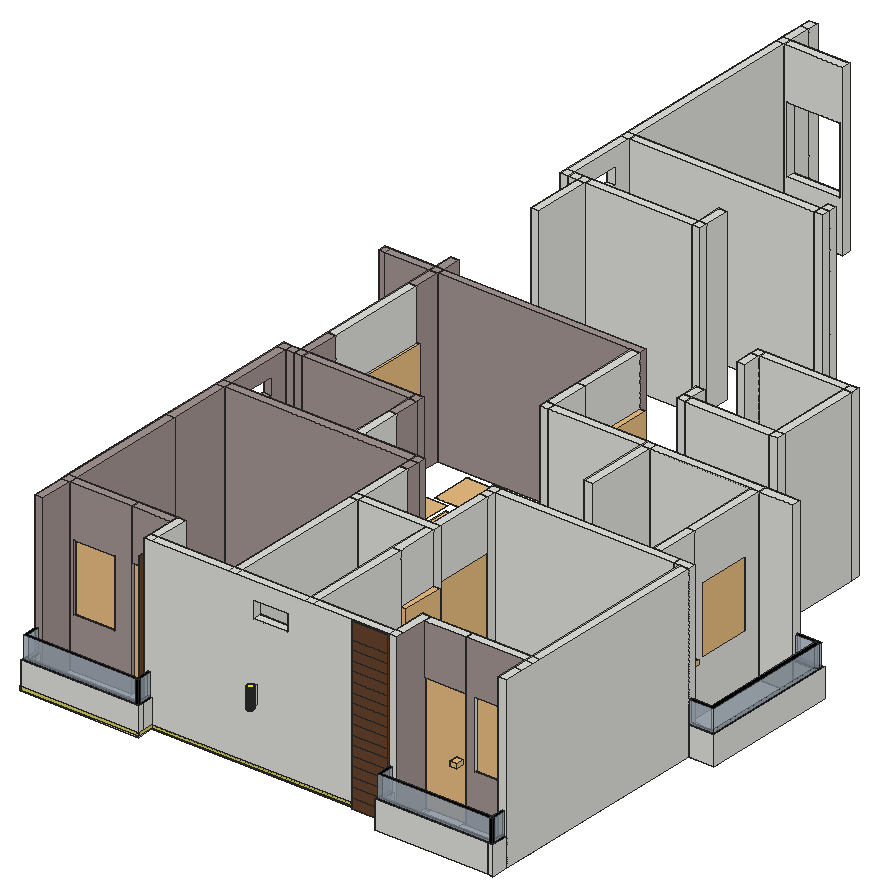
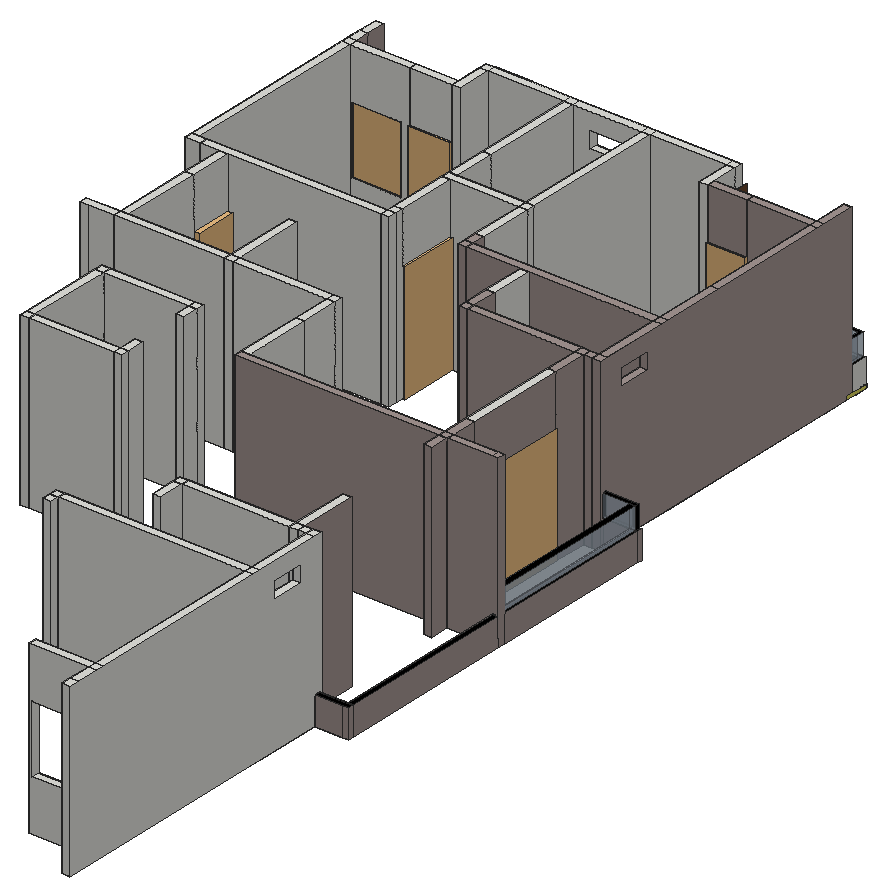
# SketchUp Ruby script. Lengths in inches.
U = 1.inch
M = Sketchup.active_model
def pt(a) = Geom::Point3d.new(a.map { |v| v * U })
def face(e, loops, mat)
  f = e.add_face(loops[0].map { |a| pt(a) })
  loops[1..].each { |l| e.add_face(l.map { |a| pt(a) }).erase! }
  f.material = f.back_material = mat if mat
  f
end
# faces: each face lists its corners as indices into pts; further lists are holes
def faces(e, pts, list, mat = nil) = list.each { |f| face(e, (f[0].is_a?(Array) ? f : [f]).map { |l| l.map { |i| pts[i] } }, mat) }
# xy, xz, yz: faces in a plane at the given z, y or x. An outline is a flat list of corners, or four numbers for a rectangle; further outlines are holes
def ring(l) = l.size == 4 ? [[l[0], l[1]], [l[2], l[1]], [l[2], l[3]], [l[0], l[3]]] : l.each_slice(2).to_a
def flat(e, list, mat, &to3) = list.each { |f| face(e, (f[0].is_a?(Array) ? f : [f]).map { |l| ring(l).map { |u, v| to3.(u, v) } }, mat) }
def xy(e, z, list, mat = nil) = flat(e, list, mat) { |x, y| [x, y, z] }
def xz(e, y, list, mat = nil) = flat(e, list, mat) { |x, z| [x, y, z] }
def yz(e, x, list, mat = nil) = flat(e, list, mat) { |y, z| [x, y, z] }
def lines(e, pts, list) = list.each { |a, b| e.add_line(pt(pts[a]), pt(pts[b])) }
# prism: a flat outline (further loops are holes) pulled along v
def prism(e, loops, v, mat = nil)
  f = face(e, loops, mat); d = Geom::Vector3d.new(v.map { |x| x * U })
  f.pushpull(f.normal.samedirection?(d) ? d.length : -d.length)
end
def box(e, o, s, mat = nil) = prism(e, [[o, [o[0] + s[0], o[1], o[2]], [o[0] + s[0], o[1] + s[1], o[2]], [o[0], o[1] + s[1], o[2]]]], [0, 0, s[2]], mat)
def at(x, y, z, deg = 0) = Geom::Transformation.translation(pt([x, y, z])) * Geom::Transformation.rotation(ORIGIN, Z_AXIS, deg.degrees)
def axes(o, x, y, z) = Geom::Transformation.new([*x, 0, *y, 0, *z, 0, *pt(o).to_a, 1])
def part(name) = M.definitions.add(name)
# library, detail: a bought-in or finely detailed component or shape, given as its bounding box
def library(name, o, s) = part(name).tap { |d| box(d.entities, o, s) }
def detail(e, o, s) = box(e.add_group.entities, o, s)
def put(e, d, t, mat = nil) = e.add_instance(d, t).tap { |i| i.material = mat if mat }
def group(e, t, mat = nil) = e.add_group.tap { |g| g.transformation = t; g.material = mat if mat }.entities
root = M.entities
M.materials.add("2121 AP  X165 Dhaani-I").color = [217, 210, 92]
M.materials.add("Glass_Basic_01").color = [161, 173, 186]
M.materials["Glass_Basic_01"].alpha = 0.59
M.materials.add("M09_Shadow_Night").color = [0, 0, 0]
M.materials.add("Marble_06_1K").color = [165, 150, 147]
M.materials.add("Wood_Veneer_15_1K").color = [103, 69, 45]
M.materials.add("[0056_Yellow]").color = [255, 255, 0]
c1 = part("Group\#8")
xy(c1.entities,0,[[0,-8.88,4,-4.88],[4,-8.88,80,-4.88],[80,-8.88,84,-4.88],[0,-4.88,4,0],[80,-4.88,84,3.12],
  [0,0,4,3.12]])
xy(c1.entities,20,[[0,-8.88,4,-4.88],[4,-8.88,80,-4.88],[80,-8.88,84,-4.88],[0,-4.88,4,0],[80,-4.88,84,3.12],
  [0,0,4,3.12]],"M09_Shadow_Night")
xz(c1.entities,-8.88,[[0,0,80,20],[80,0,84,20]])
xz(c1.entities,-4.88,[[4,0,80,20]])
xz(c1.entities,3.12,[[0,0,4,20],[80,0,84,20]])
yz(c1.entities,0,[[-8.88,0,3.12,20]])
yz(c1.entities,4,[[-4.88,0,0,20],[0,0,3.12,20]])
yz(c1.entities,80,[[-8.88,0,-4.88,20],[-4.88,0,3.12,20]])
yz(c1.entities,84,[[-8.88,0,3.12,20]])
c2 = part("Group\#6")
xy(c2.entities,0,[[0,-8,80,-4],[80,-8,84,-4],[0,-4,4,0],[80,-4,84,4],[0,0,4,4]])
xy(c2.entities,20,[[0,-8,84,-8,84,4,80,4,80,-4,4,-4,4,4,0,4]],"M09_Shadow_Night")
xz(c2.entities,-8,[[0,0,84,20]])
xz(c2.entities,-4,[[4,0,80,20]])
xz(c2.entities,4,[[0,0,4,20],[80,0,84,20]])
yz(c2.entities,0,[[-8,0,4,20]])
yz(c2.entities,4,[[-4,0,0,20],[0,0,4,20]])
yz(c2.entities,80,[[-4,0,4,20]])
yz(c2.entities,84,[[-8,0,-4,20],[-4,0,4,20]])
c3 = part("Group\#87")
xy(c3.entities,0,[[0,0,0,11.0625,2,11.0625,2,2,80,2,80,0],[80,0,82,2],[80,2,82,11.0625]])
xy(c3.entities,16,[[0,0,80,0,80,2,2,2,2,11.0625,0,11.0625],[80,0,82,2],[80,2,82,11.0625]],"M09_Shadow_Night")
xz(c3.entities,0,[[0,0,80,16]],"Glass_Basic_01")
xz(c3.entities,0,[[80,0,82,16]],"M09_Shadow_Night")
xz(c3.entities,2,[[2,0,80,16],[80,0,82,16]])
xz(c3.entities,11.0625,[[0,0,2,16],[80,0,82,16]])
yz(c3.entities,0,[[0,0,11.0625,16]])
yz(c3.entities,2,[[2,0,11.0625,16]])
yz(c3.entities,80,[[0,0,2,16],[2,0,11.0625,16]])
yz(c3.entities,82,[[2,0,11.0625,16]])
yz(c3.entities,82,[[0,0,2,16]],"M09_Shadow_Night")
c4 = part("Group\#89")
xy(c4.entities,0,[[0,0,0,11.0625,2,11.0625,2,2,80,2,80,0],[80,0,82,2],[80,2,82,11.0625]])
xy(c4.entities,16,[[0,0,80,0,80,2,2,2,2,11.0625,0,11.0625],[80,0,82,2],[80,2,82,11.0625]],"M09_Shadow_Night")
xz(c4.entities,0,[[0,0,80,16]],"Glass_Basic_01")
xz(c4.entities,0,[[80,0,82,16]],"M09_Shadow_Night")
xz(c4.entities,2,[[2,0,80,16],[80,0,82,16]])
xz(c4.entities,11.0625,[[0,0,2,16],[80,0,82,16]])
yz(c4.entities,0,[[0,0,11.0625,16]])
yz(c4.entities,2,[[2,0,11.0625,16]])
yz(c4.entities,80,[[0,0,2,16],[2,0,11.0625,16]])
yz(c4.entities,82,[[2,0,11.0625,16]])
yz(c4.entities,82,[[0,0,2,16]],"M09_Shadow_Night")
c5 = part("Wall light")
xy(c5.entities,0,[[1.3,1.93,0.875,2.1,0.51,2.38,0.23,2.74,0.06,3.17,0,3.62,0.06,4.07,0.23,4.49,0.51,4.86,0.875,5.13,1.3,5.31,1.75,5.37,2.2,5.31,2.625,5.13,2.99,4.86,3.27,4.49,3.44,4.07,3.5,3.62,3.44,3.17,3.27,2.74,2.99,2.38,2.625,2.1,2.2,1.93]],"[0056_Yellow]")
xy(c5.entities,0.74,[[1.01,0,2.57,1.93]])
xy(c5.entities,10.13,[[1.01,0,2.57,0,2.57,1.93,2.2,1.93,1.75,1.87,1.3,1.93,1.01,1.93]])
xy(c5.entities,10.875,[[1.75,1.87,2.2,1.93,1.3,1.93]])
xy(c5.entities,10.875,[[1.3,1.93,2.2,1.93,2.625,2.1,2.99,2.38,3.27,2.74,3.44,3.17,3.5,3.62,3.44,4.07,3.27,4.49,2.99,4.86,2.625,5.13,2.2,5.31,1.75,5.37,1.3,5.31,0.875,5.13,0.51,4.86,0.23,4.49,0.06,4.07,0,3.62,0.06,3.17,0.23,2.74,0.51,2.38,0.875,2.1]],"[0056_Yellow]")
xz(c5.entities,0,[[1.01,0.74,2.57,10.13]])
xz(c5.entities,1.93,[[1.3,0,2.2,0.74],[1.01,0.74,1.3,10.13],[1.3,0.74,2.2,10.875],[2.2,0.74,2.57,10.13]])
yz(c5.entities,1.01,[[0,0.74,1.93,10.13]])
yz(c5.entities,2.57,[[0,0.74,1.93,10.13]])
p = [[1.3,1.93,10.875],[0.875,2.1,10.875],[0.875,2.1,0],[1.3,1.93,0],[1.3,1.93,0.74],[1.3,1.93,10.13],
  [2.625,2.1,10.875],[2.2,1.93,10.875],[2.2,1.93,10.13],[2.2,1.93,0.74],[2.2,1.93,0],[2.625,2.1,0],
  [0.51,2.38,10.875],[0.51,2.38,0],[2.99,2.38,10.875],[2.99,2.38,0],[0.23,2.74,10.875],[0.23,2.74,0],
  [3.27,2.74,10.875],[3.27,2.74,0],[0.06,3.17,10.875],[0.06,3.17,0],[3.44,3.17,10.875],[3.44,3.17,0],
  [0,3.62,10.875],[0,3.62,0],[3.5,3.62,10.875],[3.5,3.62,0],[0.06,4.07,10.875],[0.06,4.07,0],
  [3.44,4.07,10.875],[3.44,4.07,0],[0.23,4.49,10.875],[0.23,4.49,0],[3.27,4.49,10.875],[3.27,4.49,0],
  [0.51,4.86,10.875],[0.51,4.86,0],[2.99,4.86,10.875],[2.99,4.86,0],[0.875,5.13,10.875],[0.875,5.13,0],
  [2.625,5.13,10.875],[2.625,5.13,0],[1.3,5.31,10.875],[1.3,5.31,0],[2.2,5.31,10.875],[2.2,5.31,0],
  [1.75,5.37,10.875],[1.75,5.37,0],[1.75,1.87,10.875],[1.75,1.87,10.13]]
faces(c5.entities,p,[[0,1,2,3,4,5],[6,7,8,9,10,11],[1,12,13,2],[14,6,11,15],[12,16,17,13],[18,14,15,19],[16,20,21,17],[22,18,19,23],
  [20,24,25,21],[26,22,23,27],[24,28,29,25],[30,26,27,31],[28,32,33,29],[34,30,31,35],[32,36,37,33],[38,34,35,39],
  [36,40,41,37],[42,38,39,43],[40,44,45,41],[46,42,43,47],[44,48,49,45],[48,46,47,49],[50,0,5,51],[7,50,51,8]])
c6 = part("Group\#144")
xy(c6.entities,0,[[0,0,84.5,0.1],[84.5,0,84.6,0.1],[0,0.1,0.5,17.21],[84.5,0.1,84.5,12.09,336.84,12.09,336.84,11.99,84.6,11.99,84.6,0.1]])
xy(c6.entities,2,[[0,0,84.5,0.1],[84.5,0,84.6,0.1],[0,0.1,0.5,17.21],[84.5,0.1,84.6,0.1,84.6,11.99,336.84,11.99,336.84,12.09,84.5,12.09]])
xz(c6.entities,0,[[0,0,84.5,2],[84.5,0,84.6,2]])
xz(c6.entities,0.1,[[0,0,0.5,2],[0.5,0,84.5,2],[84.5,0,84.6,2]])
xz(c6.entities,11.99,[[84.6,0,252.77,2],[252.77,0,336.84,2]])
xz(c6.entities,12.09,[[84.5,0,336.84,2]])
xz(c6.entities,17.21,[[0,0,0.5,2]])
yz(c6.entities,0,[[0,0,0.1,2],[0.1,0,17.21,2]])
yz(c6.entities,0.5,[[0.1,0,17.21,2]])
yz(c6.entities,84.5,[[0,0,0.1,2],[0.1,0,12.09,2]])
yz(c6.entities,84.6,[[0,0,0.1,2],[0.1,0,11.99,2]])
yz(c6.entities,336.84,[[11.99,0,12.09,2]])
c7 = library("TREE-26",[-60.96,-72.91,0],[121.92,134.74,0.01])
c8 = part("Group\#116")
xy(c8.entities,0,[[24,0,24.75,24.75]])
xy(c8.entities,107,[[24,0,24.75,24.75]])
xz(c8.entities,0,[[24,0,24.75,107]])
xz(c8.entities,24.75,[[24,0,24.75,107]])
yz(c8.entities,24,[[0,0,24.75,6],[0,6,24.75,12],[0,12,24.75,18],[0,18,24.75,24],[0,24,24.75,30],
  [0,30,24.75,36],[0,36,24.75,42],[0,42,24.75,48],[0,48,24.75,54],[0,54,24.75,60],
  [0,60,24.75,66],[0,66,24.75,72],[0,72,24.75,78],[0,78,24.75,84],[0,84,24.75,90],
  [0,90,24.75,96],[0,96,24.75,107]],"Wood_Veneer_15_1K")
yz(c8.entities,24.75,[[0,0,24.75,107]])
c9 = part("tgr")
p = [[-2.37,-3.35,0],[-2.37,-2.82,0],[-2.73,-2.82,0],[-2.73,-2.68,0],[-3.71,-2.68,0],[-3.71,-3.35,0],
  [-2.37,3.35,0],[-2.37,2.82,0],[-2.73,2.82,0],[-2.73,2.68,0],[-3.71,2.68,0],[-3.71,3.35,0],
  [3.71,-2.82,0],[-2.37,-2.46,0],[3.71,-2.46,0],[3.7,-2.46,0],[3.63,-2.07,0],[3.53,-1.68,0],
  [3.41,-1.3,0],[3.27,-0.93,0],[3.1,-0.57,0],[2.91,-0.22,0],[2.7,0.12,0],[2.46,0.4375,0],
  [2.21,0.74,0],[1.93,1.03,0],[1.64,1.3,0],[1.33,1.55,0],[1.01,1.79,0],[0.67,1.99,0],
  [0.32,2.18,0],[-0.04,2.35,0],[-0.41,2.49,0],[-0.8,2.6,0],[-1.18,2.69,0],[-1.58,2.76,0],
  [-1.97,2.8,0]]
lines(c9.entities,p,[[0,1],[1,2],[2,3],[3,4],[4,5],[5,0],[6,7],[7,8],[8,9],[9,10],[10,11],[11,6],
  [1,12],[13,14],[1,13],[12,14],[15,16],[16,17],[17,18],[18,19],[19,20],[20,21],[21,22],[22,23],
  [23,24],[24,25],[25,26],[26,27],[27,28],[28,29],[29,30],[30,31],[31,32],[32,33],[33,34],[34,35],
  [35,36],[36,7]])
c10 = library("Component\#2",[1075.72,38.58,0],[54,24,0.01])
c11 = library("Component\#1",[961.32,38.58,0],[54,24,0.01])
c12 = library("ghgjg",[-265.23,-341.01,0],[530.46,682.02,0.01])
c13 = library("Group\#52",[0,0,0],[4.66,6.14,3.22])
c14 = library("Slide Window 5'",[0,-2.02,0],[60,2.02,54])
c15 = library("Group\#51",[0,0,0],[6.9375,42,86.5])
c16 = part("GTGTGYHYHYHY")
p = [[-3.29,3.76,0],[3.29,3.76,0],[3.29,-3.76,0],[-3.29,-3.76,0]]
lines(c16.entities,p,[[0,1],[1,2],[2,3],[3,0],[0,2],[1,3]])
c17 = part("G5GTGTGT")
p = [[0.52,4.97,0],[0.52,-4.97,0],[0.36,-4.97,0],[0.36,4.97,0],[-0.08,-4.53,0],[-0.08,4.53,0],
  [0.33,4.97,0],[0.3,4.97,0],[0.28,4.96,0],[0.25,4.96,0],[0.22,4.95,0],[0.2,4.94,0],
  [0.17,4.93,0],[0.15,4.92,0],[0.12,4.9,0],[0.1,4.89,0],[0.08,4.87,0],[0.06,4.85,0],
  [0.04,4.83,0],[0.02,4.8125,0],[0,4.79,0],[-0.01,4.77,0],[-0.03,4.74,0],[-0.04,4.72,0],
  [-0.05,4.69,0],[-0.0625,4.67,0],[-0.07,4.64,0],[-0.08,4.61,0],[-0.08,4.59,0],[-0.08,4.56,0],
  [-0.08,-4.56,0],[-0.08,-4.59,0],[-0.08,-4.61,0],[-0.07,-4.64,0],[-0.0625,-4.67,0],[-0.05,-4.69,0],
  [-0.04,-4.72,0],[-0.03,-4.74,0],[-0.01,-4.77,0],[0,-4.79,0],[0.02,-4.8125,0],[0.04,-4.83,0],
  [0.06,-4.85,0],[0.08,-4.87,0],[0.1,-4.89,0],[0.12,-4.9,0],[0.15,-4.92,0],[0.17,-4.93,0],
  [0.2,-4.94,0],[0.22,-4.95,0],[0.25,-4.96,0],[0.28,-4.96,0],[0.3,-4.97,0],[0.33,-4.97,0],
  [-0.08,-1.38,0],[-0.52,-1.38,0],[-0.08,1.38,0],[-0.52,1.38,0]]
lines(c17.entities,p,[[0,1],[1,2],[2,3],[3,0],[4,5],[3,6],[6,7],[7,8],[8,9],[9,10],[10,11],[11,12],
  [12,13],[13,14],[14,15],[15,16],[16,17],[17,18],[18,19],[19,20],[20,21],[21,22],[22,23],[23,24],
  [24,25],[25,26],[26,27],[27,28],[28,29],[29,5],[4,30],[30,31],[31,32],[32,33],[33,34],[34,35],
  [35,36],[36,37],[37,38],[38,39],[39,40],[40,41],[41,42],[42,43],[43,44],[44,45],[45,46],[46,47],
  [47,48],[48,49],[49,50],[50,51],[51,52],[52,53],[53,2],[54,55],[56,57],[55,57]])
c18 = library("lcd-01",[-577.99,-134.75,0],[1155.98,269.5,0.01])
c19 = library("Group\#49",[0,0,0],[8.31,30,84])
c20 = library("JEEW",[-211.14,-299.86,0],[422.28,599.72,0.01])
c21 = library("double bed",[-999.9375,-1062.5,0],[1999.875,2125,0.01])
c22 = part("EGWF")
p = [[2.59,-3.49,0],[2.59,-3.09,0],[2.85,-3.09,0],[2.85,-2.99,0],[3.58,-2.99,0],[3.58,-3.49,0],
  [2.59,3.49,0],[2.59,3.09,0],[2.85,3.09,0],[2.85,2.99,0],[3.58,2.99,0],[3.58,3.49,0],
  [-3.58,-3.09,0],[2.59,-2.82,0],[-3.58,-2.82,0],[2.2,3.07,0],[1.81,3.04,0],[1.42,2.97,0],
  [1.03,2.89,0],[0.66,2.78,0],[0.29,2.64,0],[-0.07,2.48,0],[-0.42,2.3,0],[-0.76,2.1,0],
  [-1.08,1.875,0],[-1.39,1.63,0],[-1.68,1.37,0],[-1.96,1.09,0],[-2.21,0.79,0],[-2.45,0.48,0],
  [-2.67,0.15,0],[-2.86,-0.1875,0],[-3.04,-0.54,0],[-3.1875,-0.9,0],[-3.32,-1.28,0],[-3.42,-1.66,0],
  [-3.5,-2.04,0],[-3.55,-2.43,0]]
lines(c22.entities,p,[[0,1],[1,2],[2,3],[3,4],[4,5],[5,0],[6,7],[7,8],[8,9],[9,10],[10,11],[11,6],
  [1,12],[13,14],[1,13],[12,14],[7,15],[15,16],[16,17],[17,18],[18,19],[19,20],[20,21],[21,22],
  [22,23],[23,24],[24,25],[25,26],[26,27],[27,28],[28,29],[29,30],[30,31],[31,32],[32,33],[33,34],
  [34,35],[35,36],[36,37],[37,14]])
c23 = library("Group\#50",[0,0,0],[6.9375,42,86.5])
c24 = part("Group\#10")
xy(c24.entities,0,[[-133.3,-6,-127.3,0],[-133.3,0,-127.3,6],[-127.3,0,0,6],[0,0,10.7,6]])
xy(c24.entities,120,[[-133.3,-6,-127.3,0],[-133.3,0,-127.3,6],[-127.3,0,0,6],[0,0,10.7,6]])
xz(c24.entities,-6,[[-133.3,0,-127.3,120]])
xz(c24.entities,0,[[-133.3,0,-127.3,120],[-127.3,0,0,120],[0,0,10.7,120]])
xz(c24.entities,6,[[-133.3,0,-127.3,120],[-127.3,0,0,120],[0,0,10.7,120]])
yz(c24.entities,-133.3,[[-6,0,0,120],[0,0,6,120]])
yz(c24.entities,-127.3,[[-6,0,0,120],[0,0,6,120]])
yz(c24.entities,0,[[0,0,6,120]])
yz(c24.entities,10.7,[[0,0,6,120]])
c25 = part("Group\#85")
xy(c25.entities,0,[[0,0,0,11.0625,2,11.0625,2,2,80,2,80,0],[80,0,82,2],[80,2,82,11.0625]])
xy(c25.entities,16,[[0,0,80,0,80,2,2,2,2,11.0625,0,11.0625],[80,0,82,2],[80,2,82,11.0625]],"M09_Shadow_Night")
xz(c25.entities,0,[[80,0,82,16]])
xz(c25.entities,0,[[0,0,80,16]],"Glass_Basic_01")
xz(c25.entities,2,[[2,0,80,16],[80,0,82,16]])
xz(c25.entities,11.0625,[[0,0,2,16],[80,0,82,16]])
yz(c25.entities,0,[[0,0,11.0625,16]])
yz(c25.entities,2,[[2,0,11.0625,16]])
yz(c25.entities,80,[[0,0,2,16],[2,0,11.0625,16]])
yz(c25.entities,82,[[0,0,2,16],[2,0,11.0625,16]])
c26 = library("A$C72E23588",[-1177.7,-903.95,0],[2355.4,1807.9,0.01])
c27 = part("Group\#11")
xy(c27.entities,0,[[0,0,5.15,4],[5.15,0,13.95,4],[13.95,0,18,4],[13.95,4,18,93],[-30,36,-24,93],
  [-108,42,-102,93],[-180.4,93,-174.4,99],[-174.4,93,-108,99],[-108,93,-102,99],[-102,93,-24,99],
  [-24,93,-6,99],[-6,93,0,99],[0,93,13.95,99],[13.95,93,18,99],[-180.4,99,-174.4,126.21]])
xy(c27.entities,20,[[0,0,18,4],[13.95,4,18,4,18,99,0,99,0,93,13.95,93]],"M09_Shadow_Night")
xy(c27.entities,36,[[-30,42,-24,81]])
xy(c27.entities,84,[[-30,42,-24,81]])
xy(c27.entities,120,[[-30,36,-24,93],[-108,42,-102,93],[-180.4,93,-174.4,99],[-174.4,93,-108,99],[-108,93,-102,99],
  [-102,93,-24,99],[-24,93,0,99],[-180.4,99,-174.4,126.21]])
xz(c27.entities,0,[[0,0,18,20]])
xz(c27.entities,4,[[0,0,5.15,20],[5.15,0,13.95,20]])
xz(c27.entities,36,[[-30,0,-24,120]])
xz(c27.entities,42,[[-108,0,-102,120],[-30,36,-24,84]])
xz(c27.entities,81,[[-30,36,-24,84]])
xz(c27.entities,93,[[-180.4,0,-174.4,120],[-174.4,0,-108,120],[-108,0,-102,120],[-102,0,-30,120],[-30,0,-24,120],
  [-24,0,0,120],[0,0,13.95,20]])
xz(c27.entities,99,[[-180.4,0,-174.4,120],[-174.4,0,-108,120],[-108,0,-102,120],[-102,0,-24,120],[-24,0,-6,120],
  [-6,0,0,120],[0,0,18,20]])
xz(c27.entities,126.21,[[-180.4,0,-174.4,120]])
yz(c27.entities,-180.4,[[93,0,99,120],[99,0,126.21,120]])
yz(c27.entities,-174.4,[[93,0,99,120],[99,0,126.21,120]])
yz(c27.entities,-108,[[42,0,93,120],[93,0,99,120]])
yz(c27.entities,-102,[[42,0,93,120],[93,0,99,120]])
yz(c27.entities,-30,[[[36,0,93,120],[42,36,81,84]]])
yz(c27.entities,-24,[[[36,0,93,120],[42,36,81,84]],[93,0,99,120]])
yz(c27.entities,0,[[0,0,4,20],[93,0,99,20],[93,20,99,120]])
yz(c27.entities,13.95,[[4,0,93,20]])
yz(c27.entities,18,[[0,0,99,20]])
c28 = part("Group\#88")
xy(c28.entities,0,[[2,0,80,2],[80,0,82,2],[80,2,82,11.0625]])
xy(c28.entities,16,[[2,0,80,2],[80,0,82,2],[80,2,82,11.0625]],"M09_Shadow_Night")
xz(c28.entities,0,[[2,0,80,16]],"Glass_Basic_01")
xz(c28.entities,0,[[80,0,82,16]],"M09_Shadow_Night")
xz(c28.entities,2,[[2,0,80,16],[80,0,82,16]])
xz(c28.entities,11.0625,[[80,0,82,16]],"M09_Shadow_Night")
yz(c28.entities,2,[[0,0,2,16]],"M09_Shadow_Night")
yz(c28.entities,80,[[0,0,2,16],[2,0,11.0625,16]])
yz(c28.entities,82,[[2,0,11.0625,16]])
yz(c28.entities,82,[[0,0,2,16]],"M09_Shadow_Night")
c29 = library("porta correr aluminio",[0,0,0],[4.49,110.28,83.35])
c30 = library("BFGFV",[-4.32,-2.51,0],[8.64,5.02,0.01])
c31 = library("VVVV",[-3.39,-3.68,0],[6.78,7.36,0.01])
c32 = part("feeeeeeeeee")
p = [[-2.68,3.51,0],[-2.68,3.16,0],[-2.92,3.16,0],[-2.92,3.07,0],[-3.56,3.07,0],[-3.56,3.51,0],
  [-2.68,-3.51,0],[-2.68,-3.16,0],[-2.92,-3.16,0],[-2.92,-3.07,0],[-3.56,-3.07,0],[-3.56,-3.51,0],
  [3.56,3.16,0],[-2.68,2.93,0],[3.56,2.93,0],[-2.48,-3.13,0],[-2.04,-3.07,0],[-1.61,-2.98,0],
  [-1.1875,-2.86,0],[-0.77,-2.72,0],[-0.36,-2.55,0],[0.03,-2.35,0],[0.41,-2.13,0],[0.78,-1.88,0],
  [1.125,-1.62,0],[1.46,-1.32,0],[1.77,-1.01,0],[2.06,-0.68,0],[2.33,-0.33,0],[2.57,0.03,0],
  [2.79,0.42,0],[2.99,0.81,0],[3.16,1.22,0],[3.3,1.63,0],[3.41,2.06,0],[3.5,2.49,0]]
lines(c32.entities,p,[[0,1],[1,2],[2,3],[3,4],[4,5],[5,0],[6,7],[7,8],[8,9],[9,10],[10,11],[11,6],
  [1,12],[13,14],[1,13],[12,14],[8,15],[15,16],[16,17],[17,18],[18,19],[19,20],[20,21],[21,22],
  [22,23],[23,24],[24,25],[25,26],[26,27],[27,28],[28,29],[29,30],[30,31],[31,32],[32,33],[33,34],
  [34,35],[35,14]])
c33 = library("HYHHYHYHYHYHY",[-2.09,-4.54,0],[4.18,9.08,0.01])
c34 = part("Group\#53")
xy(c34.entities,0,[[-66,-66,-60,-60],[-60,-66,0,-60],[0,-66,6,-60],[-66,-60,-60,-48.73],[0,-60,6,0],
  [-66,-12.73,-60,0],[-66,0,-60,6],[-60,0,0,6],[0,0,6,6]])
xy(c34.entities,120,[[-66,-66,-60,-60],[-60,-66,0,-60],[0,-66,6,-60],[-66,-60,-60,-48.73],[0,-60,6,0],
  [-66,-12.73,-60,0],[-66,0,-60,6],[-60,0,0,6],[0,0,6,6]])
xz(c34.entities,-66,[[-66,0,-60,120],[-60,0,0,120],[0,0,6,120]])
xz(c34.entities,-60,[[-66,0,-60,120],[-60,0,0,120],[0,0,6,120]])
xz(c34.entities,-48.73,[[-66,0,-60,120]])
xz(c34.entities,-12.73,[[-66,0,-60,120]])
xz(c34.entities,0,[[-66,0,-60,120],[-60,0,0,120],[0,0,6,120]])
xz(c34.entities,6,[[-66,0,-60,120],[-60,0,0,120],[0,0,6,120]])
yz(c34.entities,-66,[[-66,0,-60,120],[-60,0,-48.73,120],[-12.73,0,0,120],[0,0,6,120]])
yz(c34.entities,-60,[[-66,0,-60,120],[-60,0,-48.73,120],[-12.73,0,0,120],[0,0,6,120]])
yz(c34.entities,0,[[-66,0,-60,120],[-60,0,0,120],[0,0,6,120]])
yz(c34.entities,6,[[-66,0,-60,120],[-60,0,0,120],[0,0,6,120]])
box(root,[76.2,73.34,204],[27.6,6,36],"Marble_06_1K")
box(root,[218.2,127.34,204],[6,30,36])
box(root,[163.8,163.34,204],[6,38.53,36])
box(root,[218.2,163.34,204],[6,42,36])
box(root,[119.8,217.34,203.9375],[6,30,36])
box(root,[332.2,217.34,204],[6,30,36])
box(root,[181.8,337.55,204],[6,48.35,36])
xy(root,120,[[109.8,55.34,163.8,79.34],[224.2,55.34,278.2,79.1]])
xy(root,204,[[284.2,73.34,314.2,79.34],[37.8,295.34,43.8,367.34]])
xy(root,240,[[284.2,73.34,314.2,79.34],[37.8,295.34,43.8,367.34]])
xz(root,73.34,[[284.2,204,314.2,240]],"Marble_06_1K")
xz(root,79.34,[[284.2,204,314.2,240]])
xz(root,295.34,[[37.8,204,43.8,240]])
xz(root,367.34,[[37.8,204,43.8,240]])
yz(root,37.8,[[295.34,204,367.34,240]],"Marble_06_1K")
yz(root,43.8,[[295.34,204,367.34,240]])
yz(root,284.2,[[73.34,204,79.34,240]])
yz(root,314.2,[[73.34,204,79.34,240]])
put(root,c1,at(278.2,46.22,120))
put(root,c2,at(25.8,45.34,120))
put(root,c3,at(26.8,38.27,140),"Glass_Basic_01")
put(root,c4,at(279.2,38.27,140),"Glass_Basic_01")
put(root,c5,axes([185.97,49.34,161],[-1.35,0,0],[0,-1.35,0],[0,0,1.35]))
put(root,c6,at(25.3,37.24,120.98),"2121 AP  X165 Dhaani-I")
put(root,c7,axes([36.72,48.3,120],[0,0.1317,0],[0.1317,0,0],[0,0,0.1317]))
put(root,c7,axes([350.625,48.65,120],[0,0.1317,0],[0.1317,0,0],[0,0,0.1317]))
put(root,c8,axes([278.2,24.59,120],[0,1,0],[-1.02586,0,0],[0,0,1.1215]),"Wood_Veneer_15_1K")
put(root,c8,axes([77.05,48.53,120.5],[1,0,0],[0,1.02586,0],[0,0,1.00467]),"Wood_Veneer_15_1K")
put(root,c9,axes([299.2,62.74,120],[0,-4.47464,0],[4.47464,0,0],[0,0,4.47464]))
put(root,c9,axes([88.8,62.74,120],[0,-4.47464,0],[-4.47464,0,0],[0,0,4.47464]))
put(root,c10,at(-851.52,16.76,120))
put(root,c11,at(-851.52,16.76,120))
put(root,c12,axes([194,68.98,120],[0.04,0,0],[0,-0.04,0],[0,0,0.04]))
put(root,c13,at(312.2,73.34,158.0625,180))
put(root,c13,at(101.8,75.06,156.64,180))
put(root,c14,axes([64.2,75.12,156],[-0.49488,0,0],[0,-1.4091,0],[0,0,0.89778]))
put(root,c14,axes([355.2,75.12,156],[-0.58385,0,0],[0,-1.4091,0],[0,0,0.88889]))
put(root,c15,axes([284.2,81,120],[0,-0.85622,0],[0.71429,0,0],[0,0,0.9711]))
put(root,c15,axes([76.2,81,120],[0,-0.85622,0],[0.65714,0,0],[0,0,0.9711]))
put(root,c16,axes([330.2,104.34,120],[0,-2.12603,0],[2.12603,0,0],[0,0,2.12603]))
g1 = group(root,at(103.8,49.34,120))
xy(g1,0,[[0,0,6,6],[6,0,60,6],[60,0,66,6],[66,0,114.4,6],[114.4,0,120.4,6],
  [120.4,0,174.4,6],[174.4,0,180.4,6],[0,6,6,30],[60,6,66,108],[114.4,6,120.4,78],
  [174.4,6,180.4,30],[60,108,66,114],[66,108,120.4,114]])
xy(g1,96,[[78,0,102.4,6]])
xy(g1,108,[[78,0,102.4,6]])
xy(g1,120,[[0,0,6,6],[6,0,60,6],[60,0,66,6],[66,0,114.4,6],[114.4,0,120.4,6],
  [120.4,0,174.4,6],[174.4,0,180.4,6],[0,6,6,30],[60,6,66,108],[114.4,6,120.4,78],
  [174.4,6,180.4,30],[60,108,66,114],[66,108,120.4,114]])
xz(g1,0,[[[0,0,180.4,120],[78,96,102.4,108]]])
xz(g1,6,[[0,0,6,120],[6,0,60,120],[60,0,66,120],[[66,0,114.4,120],[78,96,102.4,108]],[114.4,0,120.4,120],
  [120.4,0,174.4,120]])
xz(g1,30,[[0,0,6,120],[174.4,0,180.4,120]])
xz(g1,78,[[114.4,0,120.4,120]])
xz(g1,108,[[60,0,66,120],[66,0,120.4,120]])
xz(g1,114,[[60,0,66,120],[66,0,120.4,120]])
yz(g1,0,[[0,0,6,120],[6,0,30,120]])
yz(g1,6,[[6,0,30,120]])
yz(g1,60,[[6,0,108,120],[108,0,114,120]])
yz(g1,66,[[6,0,108,120],[108,0,114,120]])
yz(g1,78,[[0,96,6,108]])
yz(g1,102.4,[[0,96,6,108]])
yz(g1,114.4,[[6,0,78,120]])
yz(g1,120.4,[[6,0,78,120],[108,0,114,120]])
yz(g1,174.4,[[6,0,30,120]])
yz(g1,180.4,[[0,0,30,120]],"Marble_06_1K")
put(root,c17,axes([226.1,107.57,120],[3.62,0,0],[0,3.62,0],[0,0,3.62]))
put(root,c18,axes([158.41,128.75,120],[0,-0.04,0],[0.04,0,0],[0,0,0.04]))
g2 = group(root,at(356.2,49.34,120))
xy(g2,0,[[0,0,6,13.86],[0,13.86,6,24],[-42,24,0,30],[0,24,6,30],[0,30,6,162]])
xy(g2,36,[[-36,24,-1,30]])
xy(g2,84,[[-36,24,-1,30]])
xy(g2,120,[[0,0,6,13.86],[0,13.86,6,24],[-42,24,0,30],[0,24,6,30],[0,30,6,162]])
xz(g2,0,[[0,0,6,120]])
xz(g2,24,[[[-42,0,0,120],[-36,36,-1,84]]],"Marble_06_1K")
xz(g2,30,[[[-42,0,0,120],[-36,36,-1,84]]])
xz(g2,162,[[0,0,6,120]])
yz(g2,-42,[[24,0,30,120]])
yz(g2,-36,[[24,36,30,84]])
yz(g2,-1,[[24,36,30,84]])
yz(g2,0,[[24,0,30,120],[30,0,162,120]])
yz(g2,0,[[0,0,13.86,120],[13.86,0,24,120]],"Marble_06_1K")
yz(g2,6,[[0,0,162,120]])
put(root,c9,axes([207.6,142.34,120],[-4.47464,0,0],[0,-4.47464,0],[0,0,4.47464]))
put(root,c19,at(219.92,127.34,120))
put(root,c20,axes([178.84,144.49,120],[-0.04284,0,0],[0,0.04284,0],[0,0,0.04284]))
put(root,c21,axes([316.9375,148.2,120],[0,-0.03695,0],[0.03695,0,0],[0,0,0.03695]))
put(root,c21,axes([71.06,148.29,120],[0,-0.03695,0],[-0.03695,0,0],[0,0,0.03695]))
put(root,c19,axes([163.72,163.34,120],[1,0,0],[0,1.28434,0],[0,0,1]))
put(root,c22,axes([148.2,184.34,120],[6.02515,0,0],[0,-6.02515,0],[0,0,6.02515]))
put(root,c23,axes([216.54,163.34,120],[0.85622,0,0],[0,1,0],[0,0,0.9711]))
put(root,c22,axes([239.8,184.34,120],[-6.02515,0,0],[0,-6.02515,0],[0,0,6.02515]))
put(root,c24,at(351.5,211.34,120))
put(root,c7,axes([371.8,222.26,120],[0,0.1317,0],[0.1317,0,0],[0,0,0.1317]))
put(root,c19,axes([336.48,247.16,120],[-1,0,0],[0,-0.994,0],[0,0,1]))
put(root,c9,axes([109.2,232.34,120],[-4.47464,0,0],[0,4.47464,0],[0,0,4.47464]))
put(root,c15,axes([127.46,247.34,120],[-0.85622,0,0],[0,-0.71429,0],[0,0,0.9711]))
put(root,c9,axes([348.8,232.34,120],[4.47464,0,0],[0,4.47464,0],[0,0,4.47464]))
put(root,c12,axes([45.4375,241.34,120],[0,-0.04,0],[-0.04,0,0],[0,0,0.04]))
put(root,c13,at(336.48,245.16,156.75,-90))
put(root,c20,axes([106.95,256.29,120],[0,0.04284,0],[0.04284,0,0],[0,0,0.04284]))
put(root,c25,axes([379.2,212.34,140],[0,1.18,0],[-1.537,0,0],[0,0,1]),"Glass_Basic_01")
put(root,c26,axes([191.83,263.52,120],[0.0356,0,0],[0,-0.0356,0],[0,0,0.0356]))
put(root,c14,axes([337.02,292.34,155.33],[0,-0.65004,0],[1.4091,0,0],[0,0,0.88889]))
put(root,c27,at(362.2,211.34,120))
put(root,c7,axes([12.58,274.84,120],[0,0.1317,0],[0.1317,0,0],[0,0,0.1317]))
put(root,c18,axes([102.68,276.73,120],[0.04,0,0],[0,-0.04,0],[0,0,0.04]))
put(root,c7,axes([371.8,298.64,120],[0,0.1317,0],[0.1317,0,0],[0,0,0.1317]))
put(root,c28,axes([2.74,388.52,140],[0,-1.49,0],[2.08447,0,0],[0,0,1]),"Glass_Basic_01")
put(root,c29,axes([45.93,295.34,120.65],[-1.89519,0,0],[0,0.65291,0],[0,0,1]))
put(root,c30,axes([101.4,333.38,120],[4.3395,0,0],[0,-4.3395,0],[0,0,4.3395]))
put(root,c31,axes([64.42,333.77,120],[4.47564,0,0],[0,-4.47564,0],[0,0,4.47564]))
put(root,c31,axes([138,333.77,120],[-4.47564,0,0],[0,-4.47564,0],[0,0,4.47564]))
put(root,c32,axes([163.46,361.55,120],[-6.83664,0,0],[0,6.83664,0],[0,0,6.83664]))
put(root,c19,axes([183.52,337.55,120],[1,0,0],[0,1.6118,0],[0,0,1]))
put(root,c33,axes([99.08,366.86,120],[0,6.75189,0],[6.75189,0,0],[0,0,6.75189]))
put(root,c7,axes([12.58,379.27,120],[0,0.1317,0],[0.1317,0,0],[0,0,0.1317]))
g3 = group(root,at(25.8,731.54,120))
xy(g3,0,[[12,-255.51,18,-214.2],[0,-214.2,6,-208.2],[6,-214.2,12,-208.2],[12,-214.2,18,-208.2],[18,-214.2,94,-208.2],
  [94,-214.2,100,-208.2],[0,-208.2,6,-160.2],[94,-208.2,100,-190.2],[0,-160.2,6,-154.2],[6,-160.2,138,-154.2],
  [138,-160.2,144,-154.2],[0,-154.2,6,-116.77],[138,-154.2,144,-148.2],[0,-116.77,6,-80.17],[0,-80.17,6,-22.2],
  [0,-22.2,6,-16.2],[6,-22.2,48,-16.2],[0,-16.2,6,0],[0,0,6,7.73]])
xy(g3,36,[[8,-22.2,46,-16.2]])
xy(g3,84,[[8,-22.2,46,-16.2]])
xy(g3,96,[[0,-196.2,6,-172.2]])
xy(g3,108,[[0,-196.2,6,-172.2]])
xy(g3,120,[[12,-255.51,18,-214.2],[0,-214.2,6,-208.2],[6,-214.2,12,-208.2],[12,-214.2,18,-208.2],[18,-214.2,94,-208.2],
  [94,-214.2,100,-208.2],[0,-208.2,6,-160.2],[94,-208.2,100,-190.2],[0,-160.2,6,-154.2],[6,-160.2,138,-154.2],
  [138,-160.2,144,-154.2],[0,-154.2,6,-22.2],[138,-154.2,144,-148.2],[0,-22.2,6,-16.2],[6,-22.2,48,-16.2],
  [0,-16.2,6,0],[0,0,6,7.73]])
xz(g3,-255.51,[[12,0,18,120]])
xz(g3,-214.2,[[0,0,6,120],[6,0,12,120],[12,0,18,120],[18,0,94,120],[94,0,100,120]])
xz(g3,-208.2,[[6,0,12,120],[12,0,18,120],[18,0,94,120],[94,0,100,120]])
xz(g3,-196.2,[[0,96,6,108]])
xz(g3,-190.2,[[94,0,100,120]])
xz(g3,-172.2,[[0,96,6,108]])
xz(g3,-160.2,[[6,0,138,120],[138,0,144,120]])
xz(g3,-154.2,[[6,0,138,120],[138,0,144,120]])
xz(g3,-148.2,[[138,0,144,120]])
xz(g3,-22.2,[[[6,0,48,120],[8,36,46,84]]])
xz(g3,-16.2,[[[6,0,48,120],[8,36,46,84]]])
xz(g3,7.73,[[0,0,6,120]])
yz(g3,0,[[[-214.2,0,7.73,120],[-196.2,96,-172.2,108]]])
yz(g3,6,[[-214.2,0,-208.2,120],[[-208.2,0,-160.2,120],[-196.2,96,-172.2,108]],[-160.2,0,-154.2,120],[-154.2,0,-22.2,120],[-22.2,0,-16.2,120],
  [-16.2,0,0,120],[0,0,7.73,120]])
yz(g3,8,[[-22.2,36,-16.2,84]])
yz(g3,12,[[-214.2,0,-208.2,120]])
yz(g3,12,[[-255.51,0,-214.2,120]],"Marble_06_1K")
yz(g3,18,[[-255.51,0,-214.2,120],[-214.2,0,-208.2,120]])
yz(g3,46,[[-22.2,36,-16.2,84]])
yz(g3,48,[[-22.2,0,-16.2,120]])
yz(g3,94,[[-214.2,0,-208.2,120],[-208.2,0,-190.2,120]])
yz(g3,100,[[-214.2,0,-208.2,120],[-208.2,0,-190.2,120]])
yz(g3,138,[[-160.2,0,-154.2,120],[-154.2,0,-148.2,120]])
yz(g3,144,[[-160.2,0,-154.2,120],[-154.2,0,-148.2,120]])
g4 = group(g3,at(-2.625,-212.2,0),"Marble_06_1K")
xy(g4,0,[[2.625,-470,8.625,-446],[2.625,-446,8.625,-440],[8.625,-446,53.03,-440],[2.625,-440,8.625,-352.75],[2.625,-352.75,8.625,-308],
  [140.625,-317.47,146.625,-308],[2.625,-308,8.625,-302],[8.625,-308,140.625,-302],[140.625,-308,146.625,-302],[2.625,-302,8.625,-254],
  [96.625,-272,102.625,-254],[-21.375,-254,-17.27,-250],[-17.27,-254,2.625,-250],[2.625,-254,8.625,-250],[8.625,-254,14.625,-250],
  [14.625,-254,20.625,-250],[20.625,-254,96.625,-250],[96.625,-254,102.625,-250],[-21.375,-250,-17.27,-133.43],[2.625,-250,8.625,-248],
  [8.625,-250,14.625,-248],[14.625,-250,20.625,-248],[20.625,-250,96.625,-248],[96.625,-250,102.625,-248],[14.625,-248,20.625,-224],
  [14.625,-152,20.625,-133.43],[-21.375,-133.43,-17.27,-127.79],[-17.27,-133.43,14.625,-127.79],[14.625,-133.43,20.625,-127.79],[20.625,-133.43,164.625,-127.79],
  [-21.375,-127.79,-17.27,0],[14.625,-127.79,20.625,-114.45],[-21.375,0,-17.27,4],[-17.27,0,2.625,4]])
xy(g4,20,[[-21.375,-254,2.625,-250],[-21.375,-250,-17.27,-133.43],[-21.375,-127.79,-17.27,0],[-21.375,0,2.625,4]],"M09_Shadow_Night")
xy(g4,36,[[11.33,-446,41.03,-440]])
xy(g4,84,[[11.33,-446,41.03,-440]])
xy(g4,96,[[2.625,-290,8.625,-266]])
xy(g4,108,[[2.625,-290,8.625,-266]])
xy(g4,119.9375,[[96.625,-272,102.625,-254]])
xy(g4,120,[[2.625,-470,8.625,-446],[2.625,-446,8.625,-440],[8.625,-446,53.03,-440],[2.625,-440,8.625,-352.75],[2.625,-352.75,8.625,-308],
  [140.625,-317.47,146.625,-308],[2.625,-308,8.625,-302],[8.625,-308,140.625,-302],[140.625,-308,146.625,-302],[2.625,-302,8.625,-254],
  [2.625,-254,8.625,-248],[8.625,-254,14.625,-248],[14.625,-254,20.625,-248],[20.625,-254,96.625,-248],[96.625,-254,102.625,-248],
  [14.625,-248,20.625,-224],[14.625,-152,20.625,-133.43],[-21.375,-133.43,-17.27,-127.79],[-17.27,-133.43,14.625,-127.79],[14.625,-133.43,20.625,-127.79],
  [20.625,-133.43,164.625,-127.79],[14.625,-127.79,20.625,-114.45]])
xz(g4,-470,[[2.625,0,8.625,120]])
xz(g4,-446,[[[8.625,0,53.03,120],[11.33,36,41.03,84]]],"Marble_06_1K")
xz(g4,-440,[[[8.625,0,53.03,120],[11.33,36,41.03,84]]])
xz(g4,-317.47,[[140.625,0,146.625,120]])
xz(g4,-308,[[8.625,0,140.625,120],[140.625,0,146.625,120]])
xz(g4,-302,[[8.625,0,140.625,120],[140.625,0,146.625,120]])
xz(g4,-290,[[2.625,96,8.625,108]])
xz(g4,-272,[[96.625,0,102.625,119.9375]])
xz(g4,-266,[[2.625,96,8.625,108]])
xz(g4,-254,[[-21.375,0,-17.27,20],[-17.27,0,2.625,20],[8.625,0,14.625,120],[14.625,0,20.625,120],[20.625,0,96.625,120],
  [96.625,0,102.625,119.9375],[96.625,119.9375,102.625,120]])
xz(g4,-250,[[-21.375,0,-17.27,20],[-17.27,0,2.625,20]])
xz(g4,-248,[[2.625,0,8.625,120],[8.625,0,14.625,120],[14.625,0,20.625,120],[20.625,0,96.625,120],[96.625,0,102.625,120]])
xz(g4,-224,[[14.625,0,20.625,120]])
xz(g4,-152,[[14.625,0,20.625,120]])
xz(g4,-133.43,[[-21.375,0,-17.27,20],[-17.27,0,14.625,120],[14.625,0,20.625,120],[20.625,0,164.625,120],[-21.375,20,-17.27,120]])
xz(g4,-127.79,[[-17.27,0,-17.27,20,-21.375,20,-21.375,120,14.625,120,14.625,0],[-21.375,0,-17.27,20],[14.625,0,20.625,120],[20.625,0,164.625,120]])
xz(g4,-114.45,[[14.625,0,20.625,120]])
xz(g4,0,[[-21.375,0,-17.27,20],[-17.27,0,2.625,20]])
xz(g4,4,[[-21.375,0,-17.27,20],[-17.27,0,2.625,20]])
yz(g4,-21.375,[[-254,0,-250,20],[-250,0,-133.43,20],[-133.43,0,-127.79,120],[-127.79,0,0,20],[0,0,4,20]])
yz(g4,-17.27,[[-250,0,-133.43,20],[-127.79,0,0,20]])
yz(g4,2.625,[[[-470,0,-470,120,-248,120,-248,0,-250,0,-250,20,-254,20,-254,0],[-290,96,-266,108]],[-254,0,-250,20],[0,0,4,20]])
yz(g4,8.625,[[-446,0,-440,120],[-440,0,-352.75,120],[-352.75,0,-308,120],[-308,0,-302,120],[[-302,0,-254,120],[-290,96,-266,108]],
  [-254,0,-248,120]])
yz(g4,8.625,[[-470,0,-446,120]],"Marble_06_1K")
yz(g4,11.33,[[-446,36,-440,84]])
yz(g4,14.625,[[-254,0,-248,120],[-248,0,-224,120],[-152,0,-133.43,120],[-133.43,0,-127.79,120],[-127.79,0,-114.45,120]])
yz(g4,20.625,[[-254,0,-248,120],[-248,0,-224,120],[-152,0,-133.43,120],[-133.43,0,-127.79,120],[-127.79,0,-114.45,120]])
yz(g4,41.03,[[-446,36,-440,84]])
yz(g4,53.03,[[-446,0,-440,120]])
yz(g4,96.625,[[-272,0,-254,119.9375],[-254,0,-248,120]])
yz(g4,102.625,[[-272,0,-254,119.9375],[-254,0,-248,120]])
yz(g4,140.625,[[-317.47,0,-308,120],[-308,0,-302,120]])
yz(g4,146.625,[[-317.47,0,-308,120],[-308,0,-302,120]])
yz(g4,164.625,[[-133.43,0,-127.79,120]])
put(root,c34,at(302.2,424.34,120))
